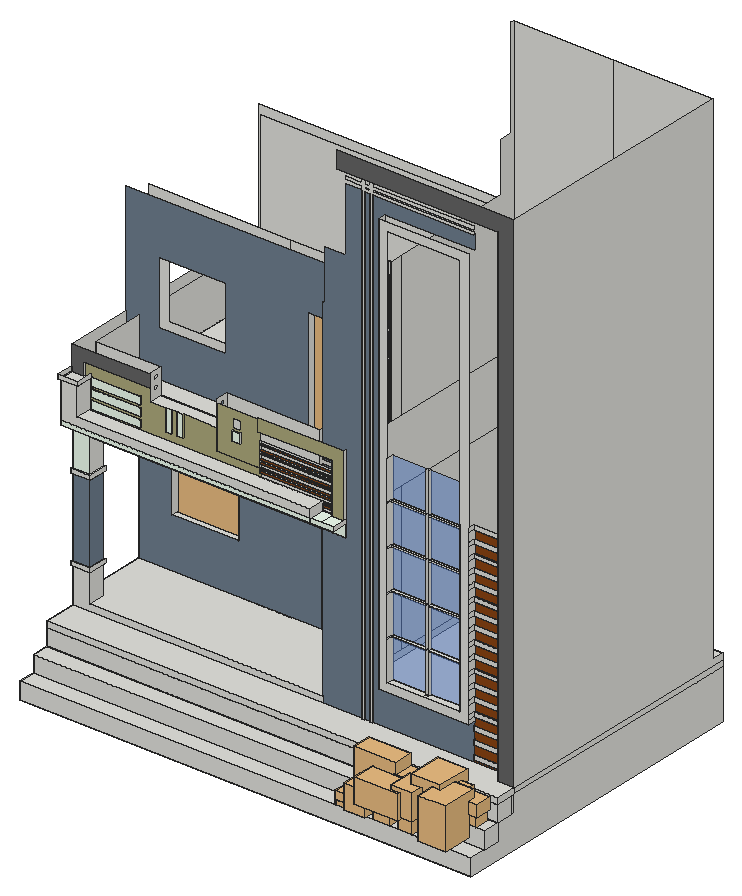
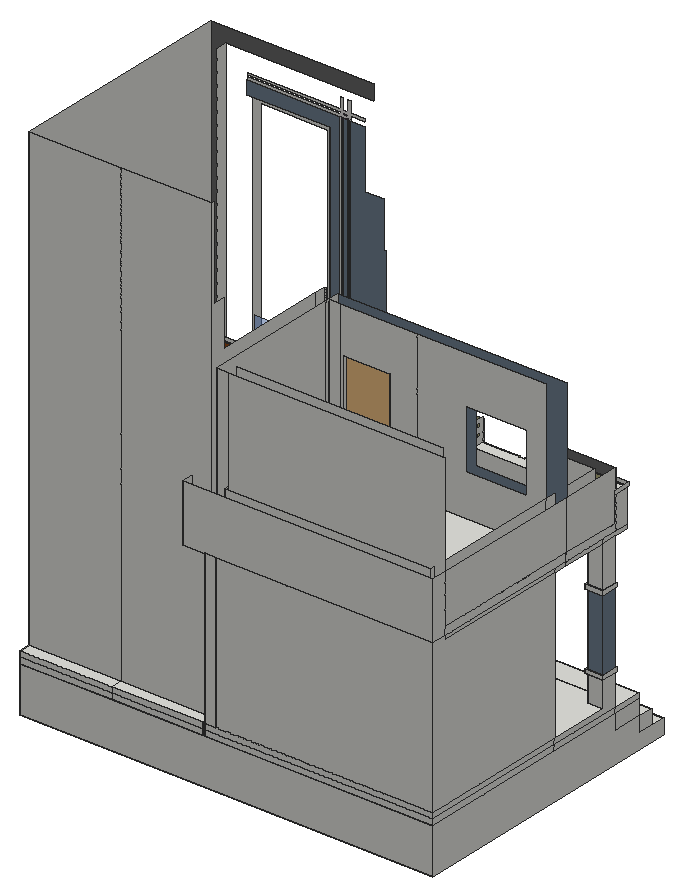
# SketchUp Ruby script. Lengths in inches.
U = 1.inch
M = Sketchup.active_model
def pt(a) = Geom::Point3d.new(a.map { |v| v * U })
def face(e, loops, mat)
  f = e.add_face(loops[0].map { |a| pt(a) })
  loops[1..].each { |l| e.add_face(l.map { |a| pt(a) }).erase! }
  f.material = f.back_material = mat if mat
  f
end
# faces: each face lists its corners as indices into pts; further lists are holes
def faces(e, pts, list, mat = nil) = list.each { |f| face(e, (f[0].is_a?(Array) ? f : [f]).map { |l| l.map { |i| pts[i] } }, mat) }
# xy, xz, yz: faces in a plane at the given z, y or x. An outline is a flat list of corners, or four numbers for a rectangle; further outlines are holes
def ring(l) = l.size == 4 ? [[l[0], l[1]], [l[2], l[1]], [l[2], l[3]], [l[0], l[3]]] : l.each_slice(2).to_a
def flat(e, list, mat, &to3) = list.each { |f| face(e, (f[0].is_a?(Array) ? f : [f]).map { |l| ring(l).map { |u, v| to3.(u, v) } }, mat) }
def xy(e, z, list, mat = nil) = flat(e, list, mat) { |x, y| [x, y, z] }
def xz(e, y, list, mat = nil) = flat(e, list, mat) { |x, z| [x, y, z] }
def yz(e, x, list, mat = nil) = flat(e, list, mat) { |y, z| [x, y, z] }
def lines(e, pts, list) = list.each { |a, b| e.add_line(pt(pts[a]), pt(pts[b])) }
# prism: a flat outline (further loops are holes) pulled along v
def prism(e, loops, v, mat = nil)
  f = face(e, loops, mat); d = Geom::Vector3d.new(v.map { |x| x * U })
  f.pushpull(f.normal.samedirection?(d) ? d.length : -d.length)
end
def box(e, o, s, mat = nil) = prism(e, [[o, [o[0] + s[0], o[1], o[2]], [o[0] + s[0], o[1] + s[1], o[2]], [o[0], o[1] + s[1], o[2]]]], [0, 0, s[2]], mat)
def at(x, y, z, deg = 0) = Geom::Transformation.translation(pt([x, y, z])) * Geom::Transformation.rotation(ORIGIN, Z_AXIS, deg.degrees)
def axes(o, x, y, z) = Geom::Transformation.new([*x, 0, *y, 0, *z, 0, *pt(o).to_a, 1])
def part(name) = M.definitions.add(name)
# library, detail: a bought-in or finely detailed component or shape, given as its bounding box
def library(name, o, s) = part(name).tap { |d| box(d.entities, o, s) }
def detail(e, o, s) = box(e.add_group.entities, o, s)
def put(e, d, t, mat = nil) = e.add_instance(d, t).tap { |i| i.material = mat if mat }
def group(e, t, mat = nil) = e.add_group.tap { |g| g.transformation = t; g.material = mat if mat }.entities
root = M.entities
M.materials.add("[0043_SaddleBrown]").color = [139, 69, 19]
M.materials.add("[0048_PaleGoldenrod]1").color = [175, 171, 125]
M.materials.add("[0066_Honeydew]").color = [240, 255, 240]
M.materials.add("[0111_SlateGray]").color = [112, 128, 144]
M.materials.add("[0134_DimGray]").color = [102, 102, 102]
M.materials.add("[Translucent Glass Blue]").color = [100, 149, 237]
M.materials["[Translucent Glass Blue]"].alpha = 0.5
c1 = library("Group232\#1",[-28.18,-36.8,18.15],[8.08,8.08,10.47])
c2 = library("Group149\#1",[30.68,-31.49,-0.01],[8.08,8.08,3.54])
c3 = library("Group169\#1",[-1.27,16.35,-0.03],[10.09,9.94,13.44])
c4 = library("Group189\#1",[32.11,-20.46,0.03],[6.45,6.35,6.15])
c5 = library("Group281\#1",[-4.5,-4.97,-0.38],[11.875,11.88,12.26])
c6 = library("Group154\#1",[29.92,-31.35,0.08],[7.87,6.92,9.03])
c7 = library("Group307\#1",[23.13,56.97,0],[5.56,5.56,8.15])
c8 = library("Group311\#1",[17.36,51.81,1.46],[15.07,16.44,16.91])
c9 = library("Group193\#1",[34.18,-25.2,3.66],[3.54,13.95,14.46])
c10 = library("Group234\#1",[-34.61,-46.7,22.37],[19.87,25.3,29.46])
c11 = library("Group283\#1",[-13.03,-11.44,9.49],[31.41,27.84,17.21])
c12 = library("Group268\#1",[32.84,-7.88,0],[6.43,7.32,5.08])
c13 = library("Group173\#1",[-3.38,12.22,11.24],[15.52,17.37,18.59])
c14 = library("Group8",[-183.25,9.15,0],[25.91,56.79,43.93])
c15 = library("Group13",[-203.48,36.63,0],[29.68,67.31,50.64])
c16 = library("Group140\#1",[24.65,23.67,0],[9.73,9.73,10.74])
c17 = library("Group181\#1",[27.96,41.23,-0.02],[8.79,8.66,7.85])
c18 = library("Group272\#1",[31.95,-9.35,4],[9.93,9.93,5.9])
c19 = library("Group176\#1",[21.13,33.45,6.91],[21.12,24.54,17.28])
c20 = library("Group276\#1",[32.34,-10.69,8.62],[12.17,13.55,12.22])
c21 = library("Group134\#1",[24.53,22.88,7.45],[11.2,11.78,8.38])
c22 = library("Group274\#1",[32.02,-9.23,9.21],[9.79,9.68,1.59])
c23 = library("Group138\#1",[24.96,24.02,9.9],[9.11,9.03,1])
c24 = library("doors",[0,-6.0625,0],[107.75,14.5625,198.25])
c25 = library("Double-hung window 69 in. x 58 in. triple row with mullions",[0,0,-2.625],[62,58,3.625])
c26 = part("Double-hung window assembly")
put(c26.entities,c25,axes([2046.74,517.98,-571.2],[-3.288,0,0],[0,0,3.072],[0,2.4,0]))
xy(root,-45,[[1,0,327,227.1875]])
xy(root,-33,[[1,0,327,12],[1,12,327,24]])
xy(root,-21,[[1,12,327,24],[1,24,1,48,210.0625,48,210.0625,47.5,212.0625,47.5,212.0625,48,215.8125,48,215.8125,47.5,217.8125,47.5,217.8125,48,315.09,48,315.09,39,327,39,327,24]])
xy(root,-9,[[1,24,327,24,327,39,315.09,39,315.09,48,217.8125,48,217.8125,47.5,215.8125,47.5,215.8125,48,212.0625,48,212.0625,47.5,210.0625,47.5,210.0625,48,1,48],[315.09,39,327,48],[210.0625,47.5,212.0625,48],[215.8125,47.5,217.8125,48],[1,48,181.625,108],
  [181.625,48,181.625,108,183,108,183,227.1875,255,227.1875,255,48],[255,48,327,227.1875],[1,108,181.375,227.1875],[181.375,108,183,227.1875]])
xy(root,-4.5,[[1,24,327,227.1875]])
xy(root,-2.85,[[291.09,47.5,315.09,48]])
xy(root,0,[[13,48,181.625,48,181.375,107.1875,169.23,107.1875,169.23,108,133.23,108,133.23,107.1875,1,107.1875,1,60,13,60],[1,107.1875,10,108],[10,107.1875,112,108],[112,107.1875,133.23,108],[169.23,107.1875,181.375,108],
  [1,108,10,227.1875],[10,108,112,116.1875],[112,108,133.23,116.1875],[133.23,108,169.23,116.1875],[169.23,108,181.375,116.1875],
  [181.375,108,183,116.1875],[10,116.1875,172.375,218.1875],[172.375,116.1875,181.375,227.1875],[181.375,116.1875,183,218.1875],[10,218.1875,112,227.1875],
  [112,218.1875,133.23,227.1875],[133.23,218.1875,169.23,227.1875],[169.23,218.1875,172.375,227.1875],[181.375,218.1875,183,227.1875],[183,218.1875,255,227.1875],
  [255,218.1875,327,227.1875]])
xy(root,0.3125,[[291.09,47.5,315.09,48]])
xy(root,6.47,[[291.09,47.5,315.09,48]])
xy(root,9.625,[[291.09,47.5,315.09,48]])
xy(root,15.78,[[291.09,47.5,315.09,48]])
xy(root,18.94,[[291.09,47.5,315.09,48]])
xy(root,21,[[0,47,14,48],[0,48,1,61],[1,48,13,60],[13,48,14,60],[1,60,14,61]])
xy(root,22.01,[[226.02,42.5,291.09,48]])
xy(root,24,[[[0,47,14,61],[1,48,13,60]],[1,48,13,60]])
xy(root,25.09,[[291.09,47.5,315.09,48]])
xy(root,28.01,[[232.02,42.5,257.55,48],[257.55,42.5,259.55,46],[259.55,42.5,285.09,48]])
xy(root,28.25,[[291.09,47.5,315.09,48]])
xy(root,34.4,[[291.09,47.5,315.09,48]])
xy(root,36,[[25,107.1875,73,116.1875]])
xy(root,37.56,[[291.09,47.5,315.09,48]])
xy(root,43.71,[[291.09,47.5,315.09,48]])
xy(root,46.87,[[291.09,47.5,315.09,48]])
xy(root,53.02,[[291.09,47.5,315.09,48]])
xy(root,56.18,[[291.09,47.5,315.09,48]])
xy(root,56.29,[[232.02,46,257.55,48],[259.55,46,285.09,48]])
xy(root,57.29,[[232.02,46,257.55,48],[259.55,46,285.09,48]])
xy(root,62.34,[[291.09,47.5,315.09,48]])
xy(root,65.49,[[291.09,47.5,315.09,48]])
xy(root,71.65,[[291.09,47.5,315.09,48]])
xy(root,74.81,[[291.09,47.5,315.09,48]])
xy(root,80.96,[[291.09,47.5,315.09,48]])
xy(root,81,[[0,47,14,48],[0,48,1,61],[1,48,13,60],[13,48,14,61],[1,60,13,61]])
xy(root,82.1875,[[25,107.1875,73,116.1875]])
xy(root,84,[[[0,47,14,61],[1,48,13,60]],[1,48,13,60],[133.23,107.1875,169.23,116.1875]])
xy(root,84.12,[[291.09,47.5,315.09,48]])
xy(root,85.57,[[232.02,46,257.55,48],[259.55,46,285.09,48]])
xy(root,86.57,[[232.02,46,257.55,48],[259.55,46,285.09,48]])
xy(root,90.27,[[291.09,47.5,315.09,48]])
xy(root,93.43,[[291.09,47.5,315.09,48]])
xy(root,99.58,[[291.09,47.5,315.09,48]])
xy(root,102.74,[[291.09,47.5,315.09,48]])
xy(root,108,[[13,48,198.375,60]])
xy(root,108.89,[[291.09,47.5,315.09,48]])
xy(root,112.05,[[291.09,47.5,315.09,48]])
xy(root,114.84,[[232.02,46,257.55,48],[259.55,46,285.09,48]])
xy(root,115.84,[[232.02,46,257.55,48],[259.55,46,285.09,48]])
xy(root,117,[[1,36.4375,181.625,48],[1,48,181.625,96.4375],[1,96.4375,181.625,215.625]])
xy(root,117,[[181.625,36.4375,198.375,48]],"[0066_Honeydew]")
xy(root,118.21,[[291.09,47.5,315.09,48]])
xy(root,120,[[189.375,45.9375,189.375,48,9.125,48,9.125,47,1,47,1,60,198.375,60,198.375,45.9375],[1,60,172.375,107.1875],[172.375,60,198.375,107.1875],[1,107.1875,172.375,107.1875,172.375,116.1875,10,116.1875,10,218.1875,172.375,218.1875,172.375,227.1875,1,227.1875],[172.375,107.1875,181.375,116.1875],
  [181.375,107.1875,198.375,116.1875],[10,116.1875,172.375,218.1875],[172.375,116.1875,181.375,227.1875],[181.375,116.1875,198.375,227.1875]])
xy(root,120,[[1,36.4375,9.125,47],[9.125,36.4375,136.36,48],[136.36,36.4375,189.375,48],[189.375,36.4375,198.375,45.9375]],"[0066_Honeydew]")
xy(root,121.36,[[291.09,47.5,315.09,48]])
xy(root,122.5,[[136.36,47.5,172.375,48],[172.375,47.5,189.375,48]])
xy(root,123.5,[[136.36,47.5,172.375,48],[172.375,47.5,189.375,48]],"[0043_SaddleBrown]")
xy(root,125,[[136.36,47.5,172.375,48],[172.375,47.5,189.375,48]])
xy(root,126,[[13,36.4375,181.375,36.4375,181.375,47.5,136.36,47.5,136.36,48,181.375,48,181.375,95.625,169.23,95.625,169.23,96.4375,133.23,96.4375,133.23,95.625,1,95.625,1,48.4375,13,48.4375],[181.375,36.4375,181.625,47.5],[136.36,47.5,172.375,48],[181.375,48,181.625,96.4375],[1,95.625,10,96.4375],
  [10,95.625,112,96.4375],[112,95.625,133.23,96.4375],[169.23,95.625,181.375,96.4375],[1,96.4375,10,215.625],[10,96.4375,112,104.625],
  [112,96.4375,133.23,104.625],[133.23,96.4375,169.23,104.625],[169.23,96.4375,181.375,104.625],[181.375,96.4375,181.625,104.625],[10,104.625,172.375,206.625],
  [172.375,104.625,181.375,215.625],[181.375,104.625,181.625,206.625],[10,206.625,112,215.625],[112,206.625,133.23,215.625],[133.23,206.625,169.23,215.625],
  [169.23,206.625,172.375,215.625],[181.375,206.625,181.625,215.625]])
xy(root,126,[[136.36,47.5,172.375,48],[172.375,47.5,181.375,48],[181.375,47.5,181.625,48],[181.625,47.5,189.375,48]],"[0043_SaddleBrown]")
xy(root,127.11,[[14.32,47.5,50.14,48]],"[0048_PaleGoldenrod]1")
xy(root,127.52,[[291.09,47.5,315.09,48]])
xy(root,128.5,[[136.36,47.5,172.375,48],[172.375,47.5,189.375,48]])
xy(root,129,[[10,57,172.375,218.1875]])
xy(root,129.5,[[136.36,47.5,172.375,48],[172.375,47.5,189.375,48]],"[0043_SaddleBrown]")
xy(root,130.68,[[291.09,47.5,315.09,48]])
xy(root,131,[[136.36,47.5,172.375,48],[172.375,47.5,189.375,48]])
xy(root,131.375,[[68.2,47.5,72.45,48],[76.51,47.5,80.76,48]],"[0048_PaleGoldenrod]1")
xy(root,131.8125,[[104.95,47.5,136.36,48]])
xy(root,132,[[136.36,47.5,172.375,48],[172.375,47.5,189.375,48]],"[0043_SaddleBrown]")
xy(root,132.61,[[14.32,47.5,50.14,48]],"[0048_PaleGoldenrod]1")
xy(root,134.5,[[136.36,47.5,172.375,48],[172.375,47.5,189.375,48]])
xy(root,134.8,[[14.32,47.5,50.14,48]],"[0048_PaleGoldenrod]1")
xy(root,135.5,[[136.36,47.5,172.375,48],[172.375,47.5,189.375,48]],"[0043_SaddleBrown]")
xy(root,136.83,[[291.09,47.5,315.09,48]])
xy(root,137,[[136.36,47.5,172.375,48],[172.375,47.5,189.375,48]])
xy(root,138,[[136.36,47.5,172.375,48],[172.375,47.5,189.375,48]],"[0043_SaddleBrown]")
xy(root,139.99,[[291.09,47.5,315.09,48]])
xy(root,140.3,[[14.32,47.5,50.14,48]],"[0048_PaleGoldenrod]1")
xy(root,140.5,[[136.36,47.5,172.375,48],[172.375,47.5,189.375,48]])
xy(root,141.5,[[136.36,47.5,172.375,48],[172.375,47.5,189.375,48]],"[0043_SaddleBrown]")
xy(root,142.05,[[14.32,47.5,50.14,48]],"[0048_PaleGoldenrod]1")
xy(root,142.64,[[116.69,47,122.32,47.5]])
xy(root,143,[[136.36,47.5,172.375,48],[172.375,47.5,189.375,48]])
xy(root,144,[[136.36,47.5,172.375,48],[172.375,47.5,189.375,48]],"[0043_SaddleBrown]")
xy(root,144.12,[[232.02,46,257.55,48],[259.55,46,285.09,48]])
xy(root,145.12,[[232.02,46,257.55,48],[259.55,46,285.09,48]])
xy(root,146.14,[[291.09,47.5,315.09,48]])
xy(root,146.5,[[136.36,47.5,172.375,48],[172.375,47.5,189.375,48]])
xy(root,146.6875,[[68.2,47.5,72.45,47.5,72.45,48,76.51,48,76.51,47.5,80.76,47.5,80.76,48,104.95,48,104.95,57,57.01,57,57.01,48,68.2,48]])
xy(root,147,[[0,35.4375,14,36.4375],[0,36.4375,1,49.4375],[1,36.4375,13,48.4375],[13,36.4375,14,48.4375],[1,48.4375,14,49.4375]])
xy(root,147.5,[[136.36,47.5,172.375,48],[172.375,47.5,189.375,48]],"[0043_SaddleBrown]")
xy(root,147.55,[[14.32,47.5,50.14,48]],"[0048_PaleGoldenrod]1")
xz(root,0,[[1,-45,327,-33]])
xz(root,12,[[1,-33,327,-21]])
xz(root,24,[[1,-33,327,-21],[1,-21,327,-9],[1,-9,327,-4.5]])
xz(root,35.4375,[[0,147,14,150]])
xz(root,36.4375,[[1,120,181.625,120,181.625,126,13,126,13,147,1,147]])
xz(root,36.4375,[[1,117,181.625,120],[181.625,117,198.375,120]],"[0066_Honeydew]")
xz(root,39,[[315.09,-21,327,-9]])
xz(root,39,[[315.09,-9,327,-9,327,363,198.375,363,198.375,351,315.09,351]],"[0134_DimGray]")
xz(root,42.5,[[[226.02,22.01,291.09,326.78],[232.02,28.01,285.09,320.78]]])
xz(root,45.9375,[[189.375,120,198.375,120,198.375,165,136.36,165,136.36,156,189.375,156]],"[0048_PaleGoldenrod]1")
xz(root,46,[[232.02,56.29,257.55,57.29],[259.55,56.29,285.09,57.29],[232.02,85.57,257.55,86.57],[259.55,85.57,285.09,86.57],[232.02,114.84,257.55,115.84],
  [259.55,114.84,285.09,115.84],[232.02,144.12,257.55,145.12],[259.55,144.12,285.09,145.12]])
xz(root,47,[[0,21,14,24],[0,81,14,84]])
xz(root,47,[[116.69,142.64,122.32,149.33]],"[0066_Honeydew]")
xz(root,47,[[1,120,9.125,120,9.125,156,57.01,156,57.01,165,1,165]],"[0134_DimGray]")
xz(root,47.5,[[210.0625,-21,212.0625,-9],[215.8125,-21,217.8125,-9],[[210.0625,-9,212.0625,-9,212.0625,337.1875,215.8125,337.1875,215.8125,-9,217.8125,-9,217.8125,337.1875,291.09,337.1875,291.09,339.1875,217.8125,339.1875,217.8125,340.5,291.09,340.5,291.09,342.5,217.8125,342.5,217.8125,351,215.8125,351,215.8125,342.5,212.0625,342.5,212.0625,351,210.0625,351,210.0625,342.5,198.375,342.5,198.375,340.5,210.0625,340.5],[212.0625,339.1875,215.8125,340.5]],[291.09,-2.85,315.09,0.3125],[291.09,6.47,315.09,9.625],
  [291.09,15.78,315.09,18.94],[291.09,25.09,315.09,28.25],[291.09,34.4,315.09,37.56],[291.09,43.71,315.09,46.87],[291.09,53.02,315.09,56.18],
  [291.09,62.34,315.09,65.49],[291.09,71.65,315.09,74.81],[291.09,80.96,315.09,84.12],[291.09,90.27,315.09,93.43],[291.09,99.58,315.09,102.74],
  [291.09,108.89,315.09,112.05],[291.09,118.21,315.09,121.36],[291.09,127.52,315.09,130.68],[291.09,136.83,315.09,139.99],[291.09,146.14,315.09,149.3]])
xz(root,47.5,[[136.36,122.5,189.375,123.5],[136.36,125,189.375,126],[136.36,128.5,189.375,129.5],[136.36,131,189.375,132],[136.36,134.5,189.375,135.5],
  [136.36,137,189.375,138],[136.36,140.5,189.375,141.5],[136.36,143,189.375,144],[136.36,146.5,189.375,147.5]],"[0043_SaddleBrown]")
xz(root,47.5,[[[104.95,131.8125,136.36,163],[116.69,150.64,122.32,157.33],[116.69,142.64,122.32,149.33]]],"[0048_PaleGoldenrod]1")
xz(root,47.5,[[14.32,127.11,50.14,132.61],[68.2,131.375,72.45,146.6875],[76.51,131.375,80.76,146.6875],[14.32,134.8,50.14,140.3],[14.32,142.05,50.14,147.55]],"[0066_Honeydew]")
xz(root,48,[[1,-21,181.625,-9],[181.625,-21,210.0625,-9],[212.0625,-21,215.8125,-9],[217.8125,-21,255,-9],[255,-21,291.09,-9],
  [291.09,-21,315.09,-9],[1,-9,181.625,-9,181.625,0,13,0,13,21,1,21],[136.36,120,181.625,122.5],[181.625,120,189.375,122.5],[136.36,123.5,181.625,125],
  [181.625,123.5,189.375,125],[136.36,126,189.375,128.5],[136.36,129.5,189.375,131],[136.36,132,189.375,134.5],[136.36,135.5,189.375,137],
  [136.36,138,189.375,140.5],[136.36,141.5,189.375,143],[136.36,144,189.375,146.5],[136.36,147.5,189.375,149]])
xz(root,48,[[291.09,-9,315.09,-2.85],[291.09,0.3125,315.09,6.47],[291.09,9.625,315.09,15.78],[291.09,18.94,315.09,25.09],[291.09,28.25,315.09,34.4],
  [291.09,37.56,315.09,43.71],[291.09,46.87,315.09,53.02],[291.09,56.18,315.09,62.34],[291.09,65.49,315.09,71.65],[291.09,74.81,315.09,80.96],
  [291.09,84.12,315.09,90.27],[291.09,93.43,315.09,99.58],[291.09,102.74,315.09,108.89],[291.09,112.05,315.09,118.21],[291.09,121.36,315.09,127.52],
  [291.09,130.68,315.09,136.83],[291.09,139.99,315.09,146.14]],"[0043_SaddleBrown]")
xz(root,48,[[[9.125,120,136.36,120,136.36,131.8125,104.95,131.8125,104.95,146.6875,80.76,146.6875,80.76,131.375,76.51,131.375,76.51,146.6875,72.45,146.6875,72.45,131.375,68.2,131.375,68.2,146.6875,57.01,146.6875,57.01,156,9.125,156],[14.32,142.05,50.14,147.55],[14.32,134.8,50.14,140.3],[14.32,127.11,50.14,132.61]]],"[0048_PaleGoldenrod]1")
xz(root,48,[[1,84,13,84,13,108,181.625,108,181.625,117,1,117],[181.625,108,198.375,117]],"[0066_Honeydew]")
xz(root,48,[[181.625,-9,210.0625,-9,210.0625,337.1875,198.375,337.1875,198.375,291,183,291,183,255,181.625,255,181.625,156,189.375,156,189.375,154,181.625,154,181.625,153,189.375,153,189.375,150,181.625,150,181.625,149,189.375,149,189.375,147.5,181.625,147.5,181.625,146.5,189.375,146.5,189.375,144,181.625,144,181.625,143,189.375,143,189.375,141.5,181.625,141.5,181.625,140.5,189.375,140.5,189.375,138,181.625,138,181.625,137,189.375,137,189.375,135.5,181.625,135.5,181.625,134.5,189.375,134.5,189.375,132,181.625,132,181.625,131,189.375,131,189.375,129.5,181.625,129.5,181.625,128.5,189.375,128.5,189.375,126,181.625,126,181.625,125,189.375,125,189.375,123.5,181.625,123.5,181.625,122.5,189.375,122.5,189.375,120,181.625,120,181.625,117,198.375,117,198.375,108,181.625,108],[212.0625,-9,215.8125,337.1875],[217.8125,-9,291.09,-9,291.09,22.01,226.02,22.01,226.02,326.78,291.09,326.78,291.09,337.1875,217.8125,337.1875],[1,24,13,81]],"[0111_SlateGray]")
xz(root,48,[[232.02,28.01,257.55,56.29],[259.55,28.01,285.09,56.29],[232.02,57.29,257.55,85.57],[259.55,57.29,285.09,85.57],[232.02,86.57,257.55,114.84],
  [259.55,86.57,285.09,114.84],[232.02,115.84,257.55,144.12],[259.55,115.84,285.09,144.12],[232.02,145.12,257.55,173.4],[259.55,145.12,285.09,173.4]],"[Translucent Glass Blue]")
xz(root,48.4375,[[1,126,13,147]])
xz(root,49.4375,[[0,147,14,150]])
xz(root,57,[[10,129,10,165,57.01,165,57.01,146.6875,104.95,146.6875,104.95,165,172.375,165,172.375,129]])
xz(root,60,[[1,0,13,21],[1,84,1,120,198.375,120,198.375,108,13,108,13,84]])
xz(root,60,[[1,24,13,81]],"[0111_SlateGray]")
xz(root,61,[[0,21,14,24],[0,81,14,84]])
xz(root,95.625,[[[1,126,133.23,126,133.23,210,169.23,210,169.23,126,181.375,126,181.375,246,1,246],[25,162,73,208.1875]]],"[0111_SlateGray]")
xz(root,96.4375,[[1,117,181.625,126]])
xz(root,104.625,[[[10,126,112,246],[25,162,73,208.1875]],[112,126,112,246,172.375,246,172.375,126,169.23,126,169.23,210,133.23,210,133.23,126],[172.375,126,181.375,246]])
xz(root,107.1875,[[[1,0,133.23,0,133.23,84,169.23,84,169.23,0,181.375,0,181.375,120,1,120],[25,36,73,82.1875]]],"[0111_SlateGray]")
xz(root,108,[[1,-9,181.375,0],[181.375,-9,181.625,0],[181.625,-9,183,0],[181.375,0,181.625,255],[181.625,0,183,255]])
xz(root,116.1875,[[[10,0,112,120],[25,36,73,82.1875]],[112,0,112,120,172.375,120,172.375,0,169.23,0,169.23,84,133.23,84,133.23,0],[172.375,0,181.375,120]])
xz(root,206.625,[[10,126,172.375,246]])
xz(root,215.625,[[1,117,181.625,126],[1,126,172.375,246],[172.375,126,181.375,246]])
xz(root,218.1875,[[10,0,172.375,120],[183,0,255,363],[255,0,327,363],[10,129,172.375,165]])
xz(root,227.1875,[[1,-45,327,-9],[1,-9,181.375,-4.5],[181.375,-9,183,-4.5],[183,-9,255,-4.5],[255,-9,327,-4.5],
  [1,-4.5,181.375,0],[181.375,-4.5,183,0],[183,-4.5,255,0],[255,-4.5,327,0],[1,0,172.375,120],
  [172.375,0,181.375,120],[1,120,198.375,165]])
yz(root,0,[[47,21,61,24],[47,81,61,84],[35.4375,147,49.4375,150]])
yz(root,1,[[0,-45,0,-33,24,-33,24,-21,48,-21,48,-9,227.1875,-9,227.1875,-45],[12,-33,24,-21],[24,-21,48,-9],[24,-9,48,-4.5],[48,-9,108,-4.5],
  [108,-9,227.1875,-4.5],[48,-4.5,48,21,60,21,60,0,108,0,108,-4.5],[108,-4.5,227.1875,0],[107.1875,0,107.1875,117,215.625,117,215.625,120,227.1875,120,227.1875,0],[48,84,60,117],
  [36.4375,117,60,120],[60,117,96.4375,120],[96.4375,117,107.1875,120],[107.1875,117,215.625,120],[36.4375,120,47,147],
  [47,120,47,147,48.4375,147,48.4375,126,96.4375,126,96.4375,120],[47,120,47,150,48.4375,150,48.4375,165,95.625,165,95.625,126,96.4375,126,96.4375,120],[96.4375,120,215.625,126],[215.625,120,227.1875,165],[95.625,126,215.625,165]])
yz(root,1,[[48,24,60,81]],"[0111_SlateGray]")
yz(root,9.125,[[47,120,48,156]])
yz(root,10,[[116.1875,0,218.1875,120],[104.625,126,206.625,129],[57,129,104.625,165],[104.625,129,206.625,165],[206.625,129,218.1875,165]])
yz(root,13,[[48,0,60,21],[48,84,60,108],[36.4375,126,48.4375,147]])
yz(root,13,[[48,24,60,81]],"[0111_SlateGray]")
yz(root,14,[[47,21,61,24],[47,81,61,84],[35.4375,147,49.4375,150]])
yz(root,14.32,[[47.5,127.11,48,132.61],[47.5,134.8,48,140.3],[47.5,142.05,48,147.55]],"[0048_PaleGoldenrod]1")
yz(root,25,[[107.1875,36,116.1875,82.1875]])
yz(root,50.14,[[47.5,127.11,48,132.61],[47.5,134.8,48,140.3],[47.5,142.05,48,147.55]],"[0048_PaleGoldenrod]1")
yz(root,57.01,[[[48,146.6875,57,165],[52.58,158.88,52.14,158.94,51.74,159.11,51.39,159.38,51.12,159.73,50.95,160.13,50.89,160.57,50.95,161.01,51.12,161.41,51.39,161.76,51.74,162.03,52.14,162.2,52.58,162.26,53.02,162.2,53.43,162.03,53.77,161.76,54.04,161.41,54.21,161.01,54.27,160.57,54.21,160.13,54.04,159.73,53.77,159.38,53.43,159.11,53.02,158.94],[52.58,152.13,52.14,152.19,51.74,152.36,51.39,152.63,51.12,152.98,50.95,153.38,50.89,153.82,50.95,154.26,51.12,154.66,51.39,155.01,51.74,155.28,52.14,155.45,52.58,155.51,53.02,155.45,53.43,155.28,53.77,155.01,54.04,154.66,54.21,154.26,54.27,153.82,54.21,153.38,54.04,152.98,53.77,152.63,53.43,152.36,53.02,152.19]]])
yz(root,68.2,[[47.5,131.375,48,146.6875]],"[0048_PaleGoldenrod]1")
yz(root,72.45,[[47.5,131.375,48,146.6875]],"[0048_PaleGoldenrod]1")
yz(root,73,[[107.1875,36,116.1875,82.1875]])
yz(root,76.51,[[47.5,131.375,48,146.6875]],"[0048_PaleGoldenrod]1")
yz(root,80.76,[[47.5,131.375,48,146.6875]],"[0048_PaleGoldenrod]1")
yz(root,104.95,[[47.5,131.8125,48,146.6875],[47.5,146.6875,48,163],[[48,146.6875,57,165],[52.58,158.88,53.02,158.94,53.43,159.11,53.77,159.38,54.04,159.73,54.21,160.13,54.27,160.57,54.21,161.01,54.04,161.41,53.77,161.76,53.43,162.03,53.02,162.2,52.58,162.26,52.14,162.2,51.74,162.03,51.39,161.76,51.12,161.41,50.95,161.01,50.89,160.57,50.95,160.13,51.12,159.73,51.39,159.38,51.74,159.11,52.14,158.94],[52.58,152.13,53.02,152.19,53.43,152.36,53.77,152.63,54.04,152.98,54.21,153.38,54.27,153.82,54.21,154.26,54.04,154.66,53.77,155.01,53.43,155.28,53.02,155.45,52.58,155.51,52.14,155.45,51.74,155.28,51.39,155.01,51.12,154.66,50.95,154.26,50.89,153.82,50.95,153.38,51.12,152.98,51.39,152.63,51.74,152.36,52.14,152.19]]])
yz(root,116.69,[[47,142.64,47.5,149.33]])
yz(root,122.32,[[47,142.64,47.5,149.33]])
yz(root,133.23,[[107.1875,0,116.1875,84],[95.625,126,104.625,210]])
yz(root,136.36,[[47.5,132,48,134.5],[47.5,135.5,48,137],[47.5,138,48,140.5],[47.5,141.5,48,143],[47.5,144,48,146.5],
  [47.5,147.5,48,149]])
yz(root,136.36,[[47.5,122.5,48,123.5],[47.5,125,48,126],[47.5,128.5,48,129.5],[47.5,131,48,131.8125]],"[0043_SaddleBrown]")
yz(root,169.23,[[107.1875,0,116.1875,84],[95.625,126,104.625,210]])
yz(root,172.375,[[116.1875,0,218.1875,120],[218.1875,0,227.1875,120],[104.625,126,206.625,129],[206.625,126,215.625,129],[57,129,104.625,165],
  [104.625,129,206.625,165],[206.625,129,215.625,165],[215.625,129,218.1875,165]])
yz(root,181.375,[[108,-9,227.1875,0],[107.1875,0,108,120],[108,0,116.1875,120],[116.1875,0,227.1875,120],[107.1875,120,108,126],
  [95.625,126,104.625,246],[104.625,126,107.1875,246],[107.1875,126,108,246],[108,126,215.625,246]])
yz(root,181.625,[[36.4375,117,48,126],[48,117,96.4375,126],[96.4375,117,108,126],[108,117,215.625,126]])
yz(root,183,[[108,-9,227.1875,0],[108,0,116.1875,255],[116.1875,0,116.1875,255,206.625,255,206.625,291,215.625,291,215.625,363,218.1875,363,218.1875,0]])
yz(root,189.375,[[45.9375,120,45.9375,156,48,156,48,154,47.5,154,47.5,153,48,153,48,150,47.5,150,47.5,149,48,149,48,147.5,47.5,147.5,47.5,146.5,48,146.5,48,144,47.5,144,47.5,143,48,143,48,141.5,47.5,141.5,47.5,140.5,48,140.5,48,138,47.5,138,47.5,137,48,137,48,135.5,47.5,135.5,47.5,134.5,48,134.5,48,132,47.5,132,47.5,131,48,131,48,129.5,47.5,129.5,47.5,128.5,48,128.5,48,126,47.5,126,47.5,125,48,125,48,123.5,47.5,123.5,47.5,122.5,48,122.5,48,120]])
yz(root,198.375,[[48,108,60,108,60,120,36.4375,120,36.4375,117,48,117],[45.9375,120,227.1875,165]])
yz(root,210.0625,[[47.5,-21,48,-9],[47.5,-9,48,337.1875]])
yz(root,212.0625,[[47.5,-21,48,-9],[47.5,-9,48,337.1875]])
yz(root,215.8125,[[47.5,-21,48,-9],[47.5,-9,48,337.1875]])
yz(root,217.8125,[[47.5,-21,48,-9],[47.5,-9,48,337.1875]])
yz(root,226.02,[[42.5,22.01,48,326.78]])
yz(root,232.02,[[42.5,28.01,48,56.29],[42.5,56.29,46,57.29],[42.5,57.29,48,85.57],[42.5,85.57,46,86.57],[42.5,86.57,48,114.84],
  [42.5,114.84,46,115.84],[42.5,115.84,48,144.12],[42.5,144.12,46,145.12],[42.5,145.12,48,173.4]])
yz(root,257.55,[[46,28.01,48,56.29],[46,57.29,48,85.57],[46,86.57,48,114.84],[46,115.84,48,144.12],[46,145.12,48,173.4]])
yz(root,259.55,[[46,28.01,48,56.29],[46,57.29,48,85.57],[46,86.57,48,114.84],[46,115.84,48,144.12],[46,145.12,48,173.4]])
yz(root,285.09,[[42.5,28.01,48,28.25],[42.5,28.25,48,34.4],[42.5,34.4,48,37.56],[42.5,37.56,48,43.71],[42.5,43.71,48,46.87],
  [42.5,46.87,48,53.02],[42.5,53.02,48,56.18],[42.5,56.18,48,56.29],[42.5,56.29,46,57.29],[42.5,57.29,48,62.34],
  [42.5,62.34,48,65.49],[42.5,65.49,48,71.65],[42.5,71.65,48,74.81],[42.5,74.81,48,80.96],[42.5,80.96,48,84.12],
  [42.5,84.12,48,85.57],[42.5,85.57,46,86.57],[42.5,86.57,48,90.27],[42.5,90.27,48,93.43],[42.5,93.43,48,99.58],
  [42.5,99.58,48,102.74],[42.5,102.74,48,108.89],[42.5,108.89,48,112.05],[42.5,112.05,48,114.84],[42.5,114.84,46,115.84],
  [42.5,115.84,48,118.21],[42.5,118.21,48,121.36],[42.5,121.36,48,127.52],[42.5,127.52,48,130.68],[42.5,130.68,48,136.83],
  [42.5,136.83,48,139.99],[42.5,139.99,48,144.12],[42.5,144.12,46,145.12],[42.5,145.12,48,146.14],[42.5,146.14,48,149.3]])
yz(root,291.09,[[47.5,-2.85,48,0.3125],[47.5,6.47,48,9.625],[47.5,15.78,48,18.94],[42.5,22.01,48,25.09],[42.5,25.09,47.5,28.25],
  [42.5,28.25,48,34.4],[42.5,34.4,47.5,37.56],[42.5,37.56,48,43.71],[42.5,43.71,47.5,46.87],[42.5,46.87,48,53.02],
  [42.5,53.02,47.5,56.18],[42.5,56.18,48,62.34],[42.5,62.34,47.5,65.49],[42.5,65.49,48,71.65],[42.5,71.65,47.5,74.81],
  [42.5,74.81,48,80.96],[42.5,80.96,47.5,84.12],[42.5,84.12,48,90.27],[42.5,90.27,47.5,93.43],[42.5,93.43,48,99.58],
  [42.5,99.58,47.5,102.74],[42.5,102.74,48,108.89],[42.5,108.89,47.5,112.05],[42.5,112.05,48,118.21],[42.5,118.21,47.5,121.36],
  [42.5,121.36,48,127.52],[42.5,127.52,47.5,130.68],[42.5,130.68,48,136.83],[42.5,136.83,47.5,139.99],[42.5,139.99,48,146.14],
  [42.5,146.14,47.5,149.3]])
yz(root,315.09,[[39,-21,48,-9],[39,-9,39,351,48,351,48,344.85,47.5,344.85,47.5,341.6875,48,341.6875,48,335.53,47.5,335.53,47.5,332.375,48,332.375,48,326.22,47.5,326.22,47.5,323.06,48,323.06,48,316.91,47.5,316.91,47.5,313.75,48,313.75,48,307.6,47.5,307.6,47.5,304.44,48,304.44,48,298.29,47.5,298.29,47.5,295.13,48,295.13,48,288.98,47.5,288.98,47.5,285.82,48,285.82,48,279.66,47.5,279.66,47.5,276.51,48,276.51,48,270.35,47.5,270.35,47.5,267.19,48,267.19,48,261.04,47.5,261.04,47.5,257.88,48,257.88,48,251.73,47.5,251.73,47.5,248.57,48,248.57,48,242.42,47.5,242.42,47.5,239.26,48,239.26,48,233.11,47.5,233.11,47.5,229.95,48,229.95,48,223.79,47.5,223.79,47.5,220.64,48,220.64,48,214.48,47.5,214.48,47.5,211.32,48,211.32,48,205.17,47.5,205.17,47.5,202.01,48,202.01,48,195.86,47.5,195.86,47.5,192.7,48,192.7,48,186.55,47.5,186.55,47.5,183.39,48,183.39,48,177.23,47.5,177.23,47.5,174.08,48,174.08,48,167.92,47.5,167.92,47.5,164.77,48,164.77,48,158.61,47.5,158.61,47.5,155.45,48,155.45,48,149.3,47.5,149.3,47.5,146.14,48,146.14,48,139.99,47.5,139.99,47.5,136.83,48,136.83,48,130.68,47.5,130.68,47.5,127.52,48,127.52,48,121.36,47.5,121.36,47.5,118.21,48,118.21,48,112.05,47.5,112.05,47.5,108.89,48,108.89,48,102.74,47.5,102.74,47.5,99.58,48,99.58,48,93.43,47.5,93.43,47.5,90.27,48,90.27,48,84.12,47.5,84.12,47.5,80.96,48,80.96,48,74.81,47.5,74.81,47.5,71.65,48,71.65,48,65.49,47.5,65.49,47.5,62.34,48,62.34,48,56.18,47.5,56.18,47.5,53.02,48,53.02,48,46.87,47.5,46.87,47.5,43.71,48,43.71,48,37.56,47.5,37.56,47.5,34.4,48,34.4,48,28.25,47.5,28.25,47.5,25.09,48,25.09,48,18.94,47.5,18.94,47.5,15.78,48,15.78,48,9.625,47.5,9.625,47.5,6.47,48,6.47,48,0.3125,47.5,0.3125,47.5,-2.85,48,-2.85,48,-9]])
yz(root,327,[[0,-45,227.1875,-45,227.1875,-9,39,-9,39,-21,24,-21,24,-33,0,-33],[12,-33,24,-21],[24,-21,36,-9],[36,-21,39,-21,39,-9,227.1875,-9,227.1875,-4.5,39,-4.5,39,-9,36,-9],[36,-21,39,-9],
  [24,-9,39,-4.5],[39,-4.5,227.1875,-4.5,227.1875,0,218.1875,0,218.1875,363,39,363]])
put(root,c1,at(330.37,37.95,-51.52))
put(root,c2,at(198.81,31.49,-32.99))
put(root,c3,at(275.52,-16.35,-32.97))
put(root,c4,at(258.71,20.46,-33.03))
put(root,c5,at(260.55,4.97,-32.62))
put(root,c6,at(198.81,31.49,-32.99))
put(root,c7,at(221.1875,-56.25,-32.21))
put(root,c8,at(221.1875,-56.25,-32.21))
put(root,c9,at(258.71,20.46,-33.03))
put(root,c10,at(330.37,37.95,-51.52))
put(root,c11,at(260.55,4.97,-32.62))
put(root,c12,at(266.47,19.8,-22.34))
put(root,c13,at(275.52,-16.35,-32.97))
put(root,c14,axes([229.39,-73.2,-21],[0,-0.53,0],[0.53,0,0],[0,0,0.53]))
put(root,c15,axes([252.96,-79.35,-21],[0,-0.5141,0],[0.28276,0,0],[0,0,0.30846]))
put(root,c16,at(286.5,-11.67,-21))
put(root,c17,at(259.04,-29.23,-20.98))
put(root,c18,at(266.47,19.8,-22.34))
put(root,c19,at(259.04,-29.23,-20.98))
put(root,c20,at(266.47,19.8,-22.34))
put(root,c21,at(286.5,-11.67,-21))
put(root,c22,at(266.47,19.8,-22.34))
put(root,c23,at(286.5,-11.67,-21))
put(root,c24,axes([133.23,113.26,0],[0.33411,0,0],[0,0.22231,0],[0,0,0.42371]))
put(root,c26,axes([-421.94,-0.73,186.75],[0.24252,0,0],[0,0.2204,0],[0,0,0.26392]))
put(root,c24,axes([133.23,101.7,126],[0.33411,0,0],[0,0.22231,0],[0,0,0.42371]))
